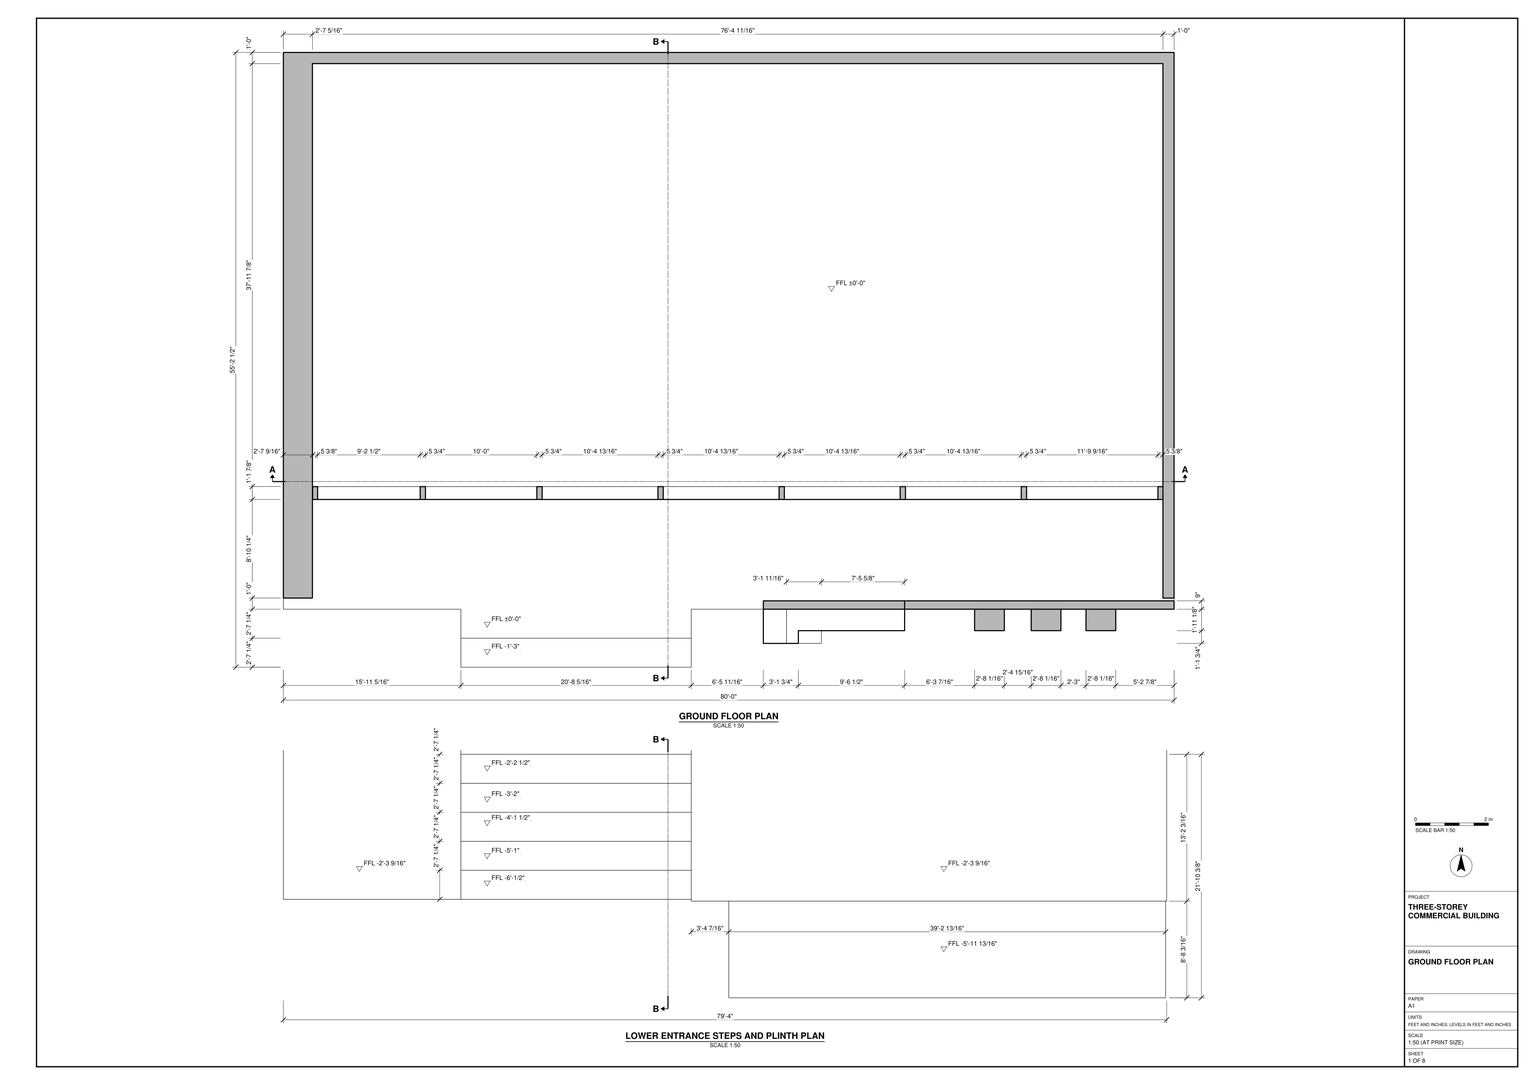
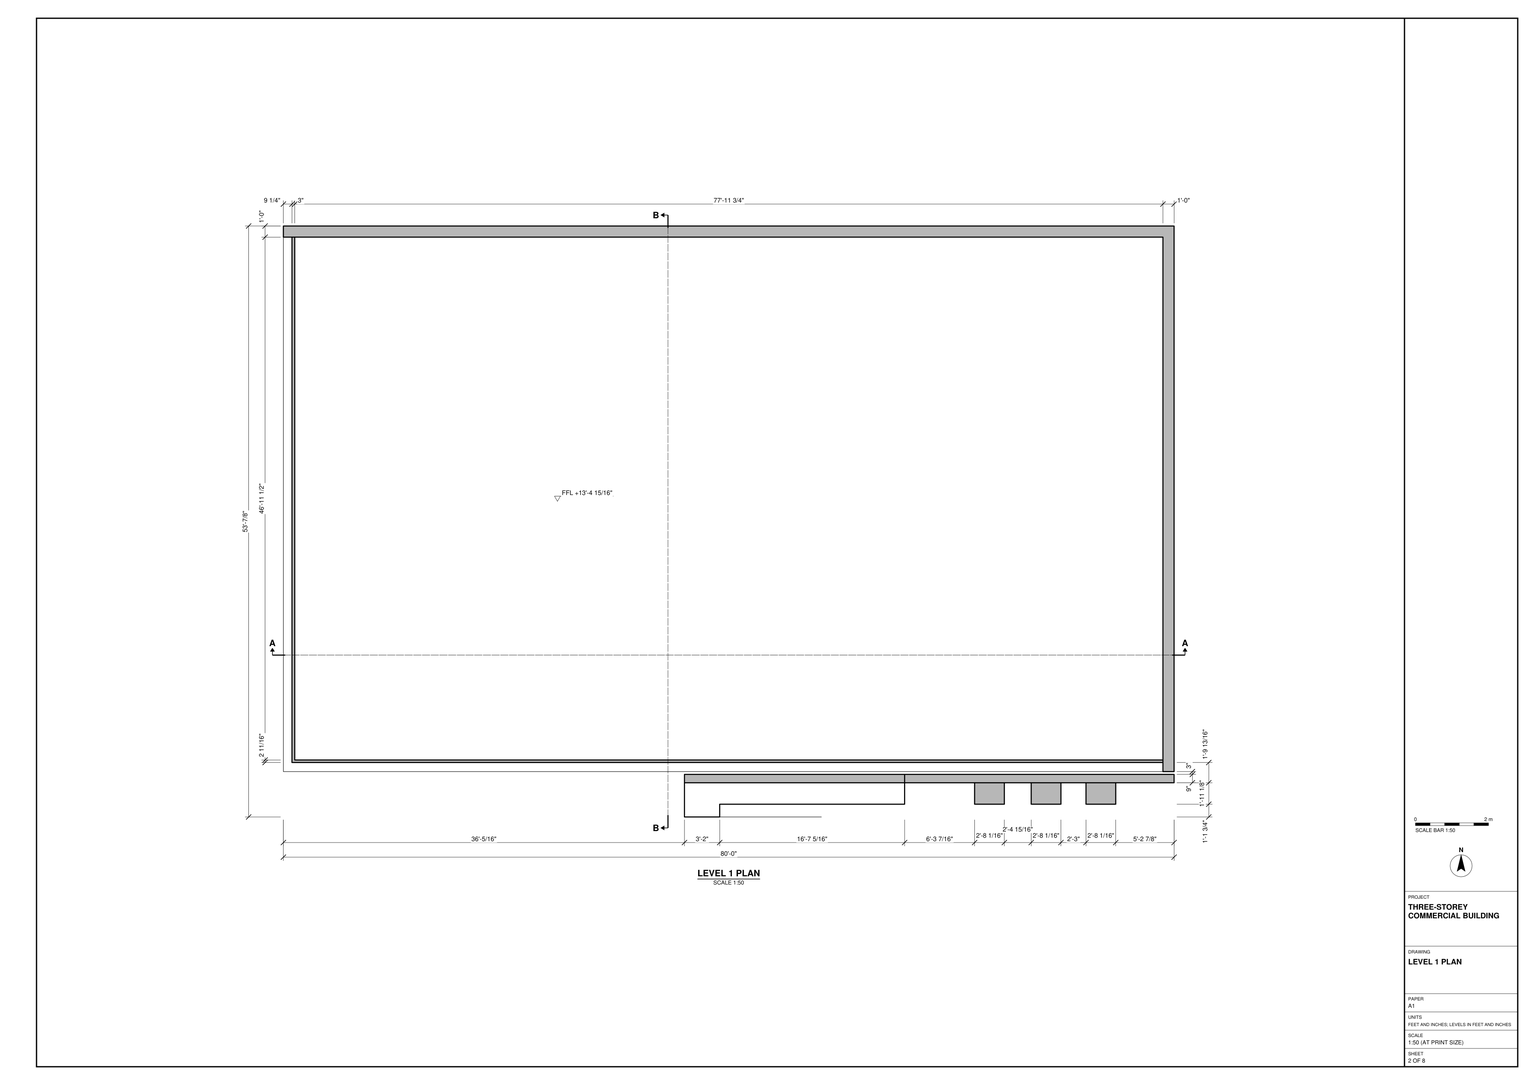
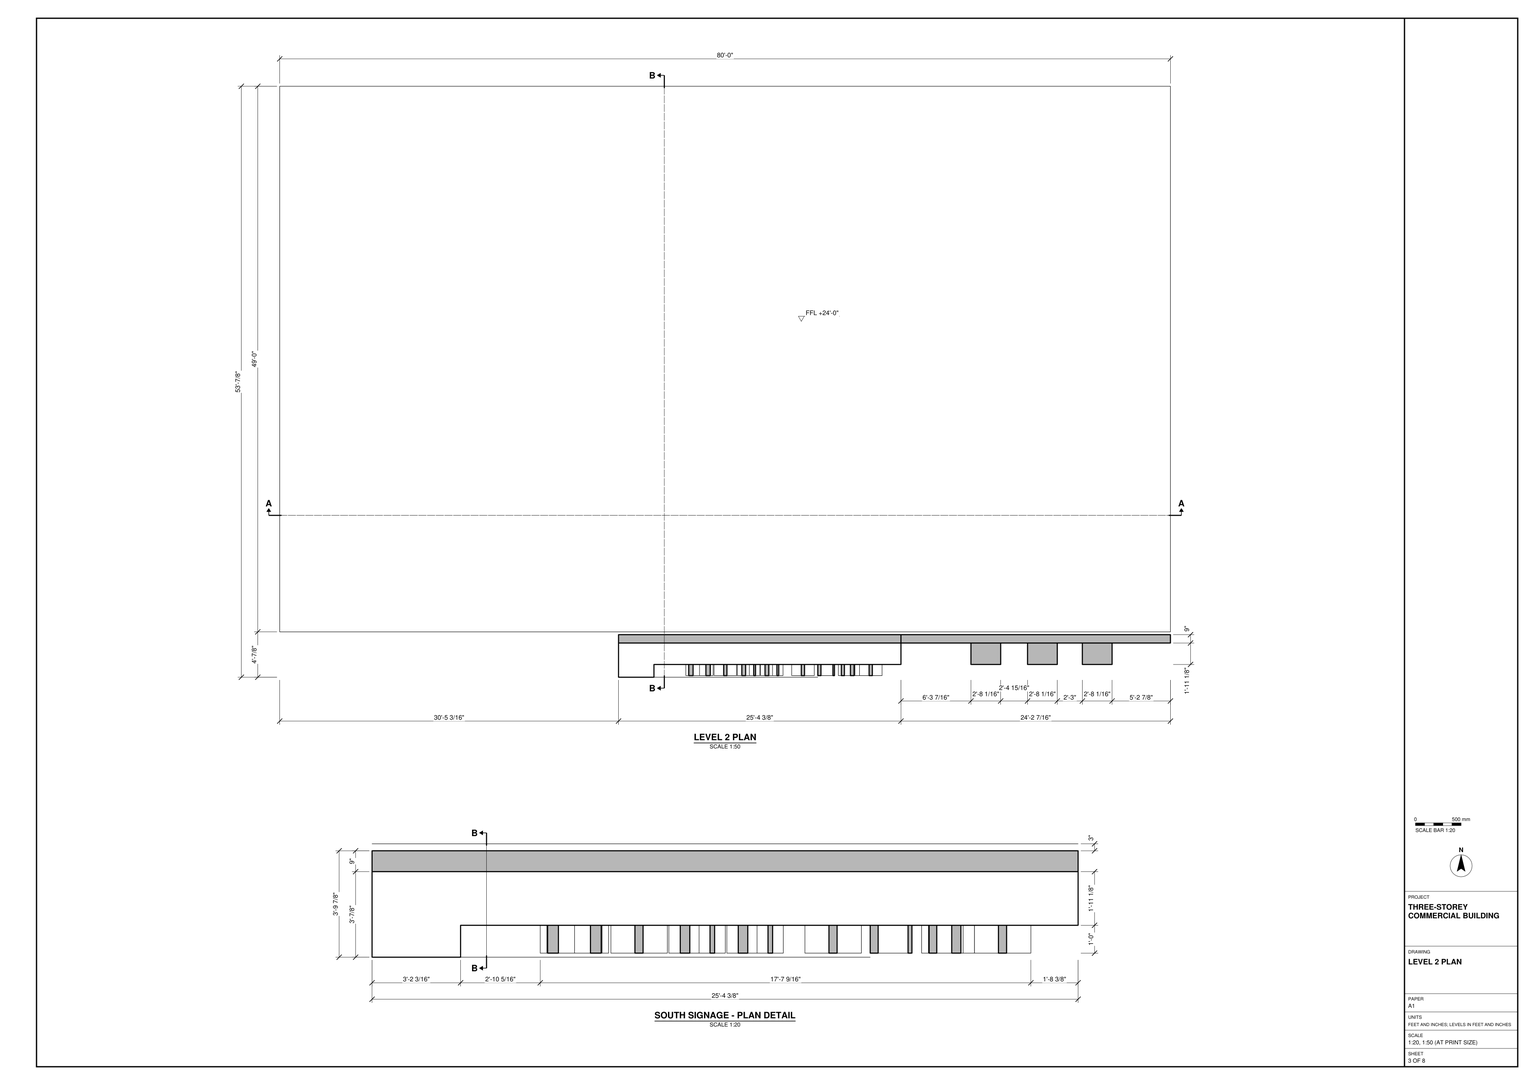
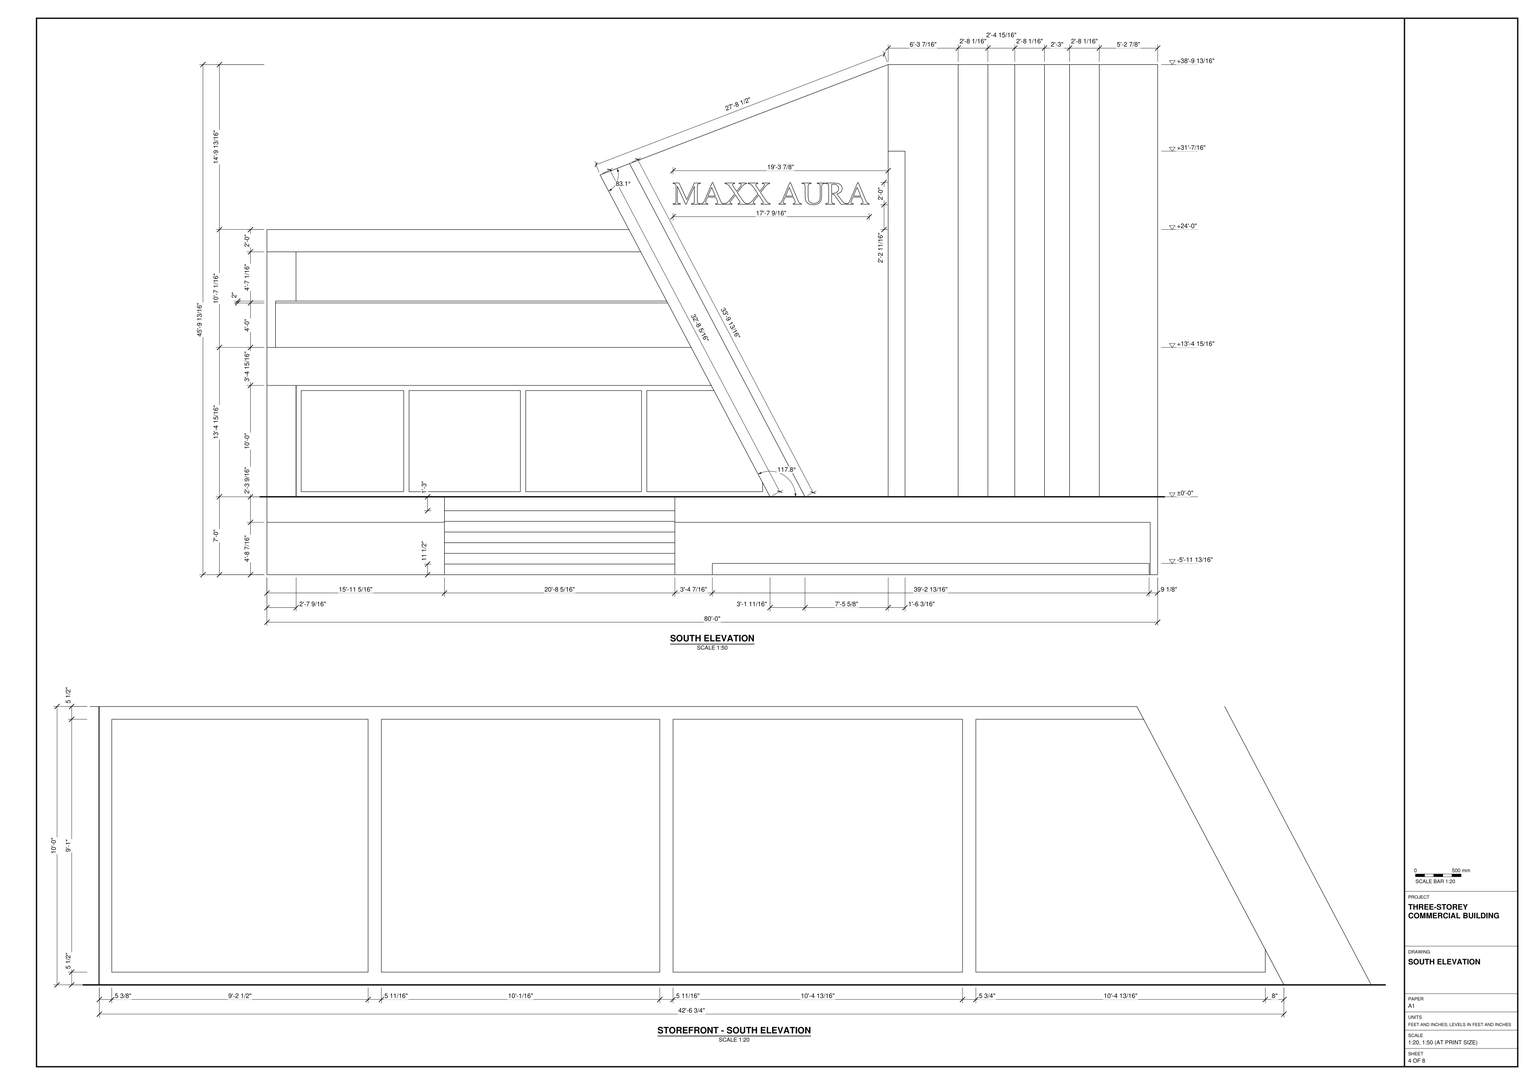
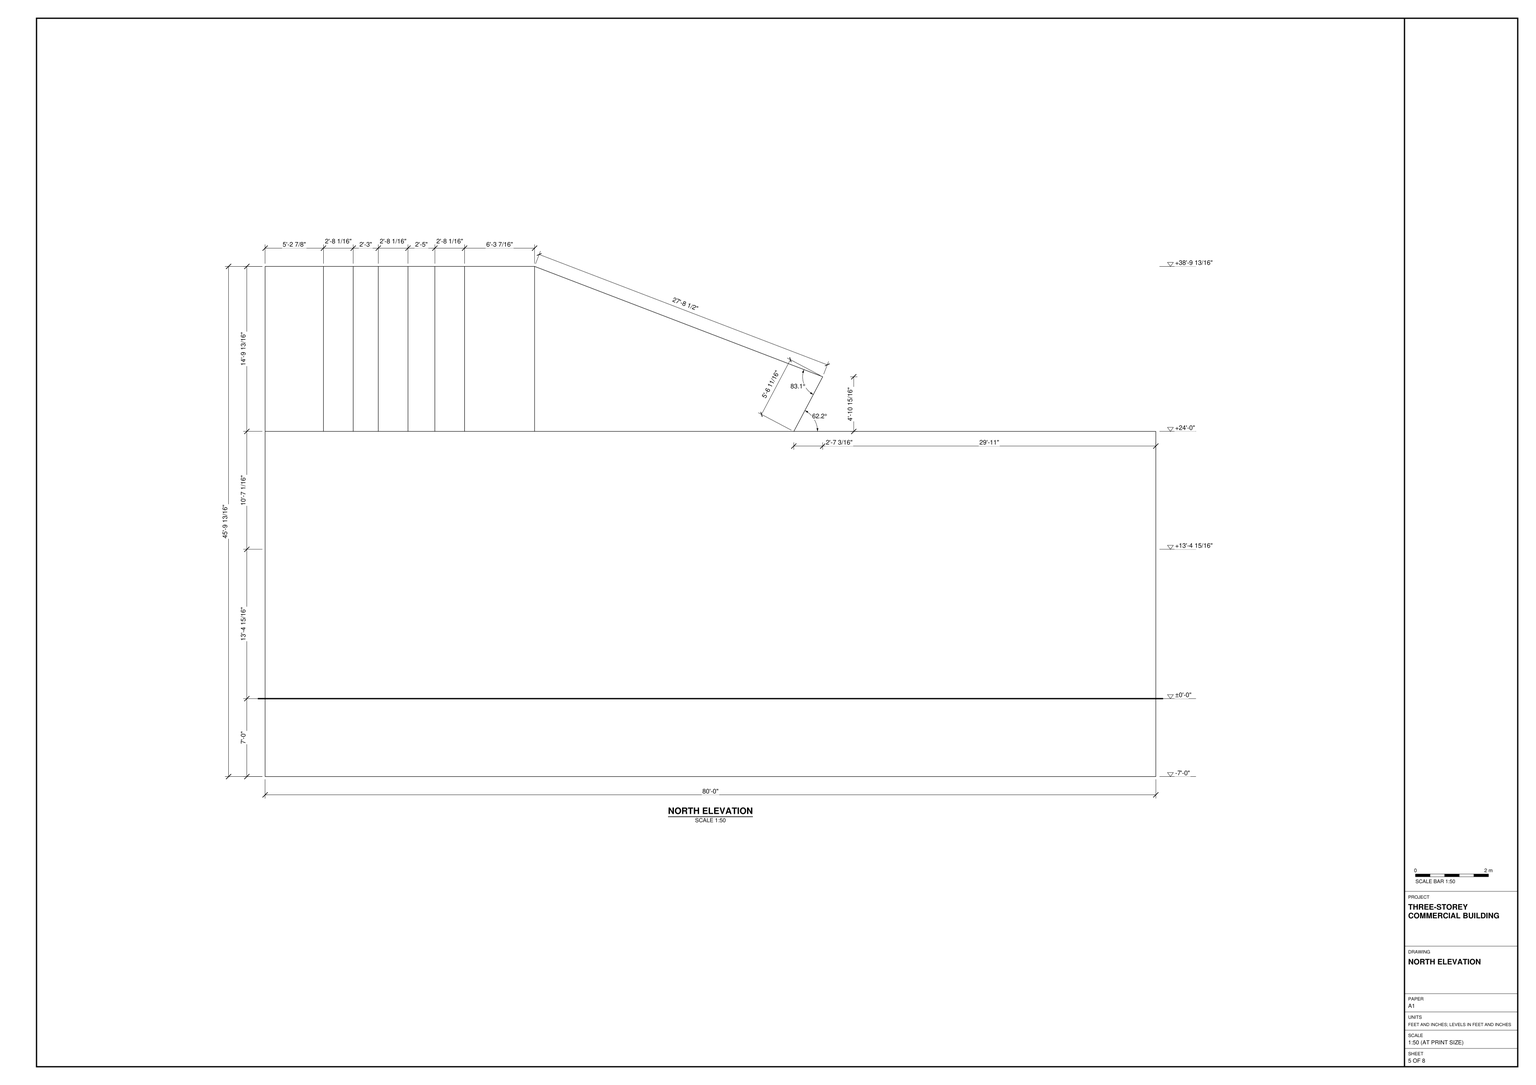
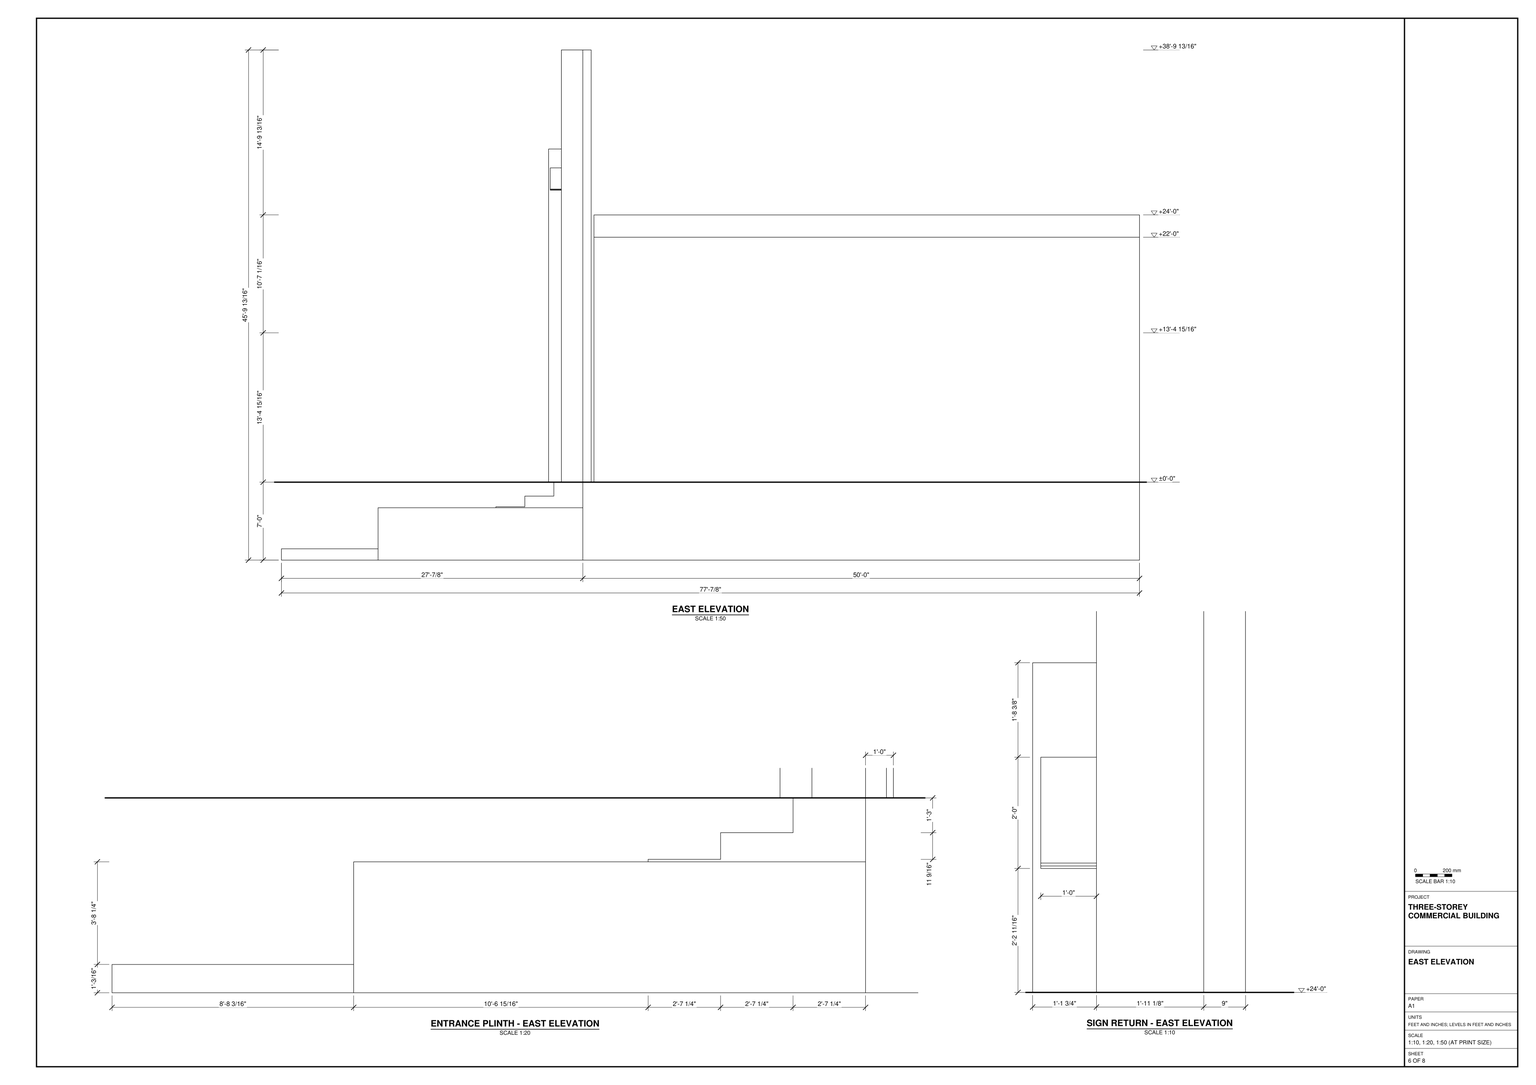
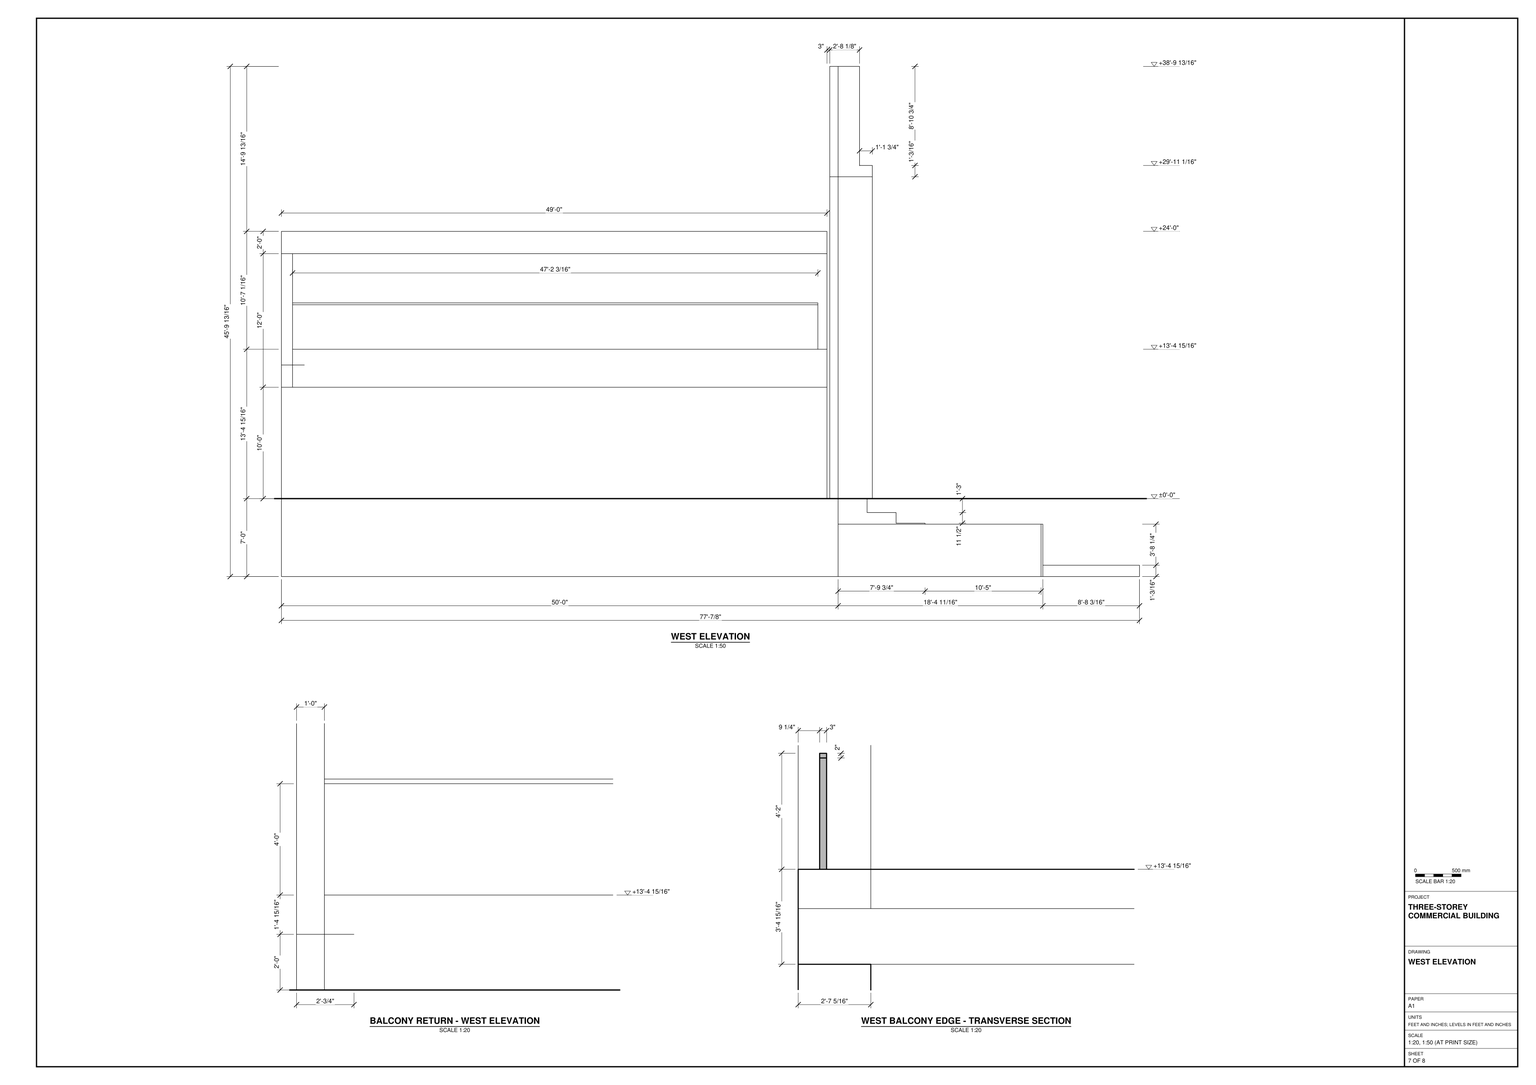
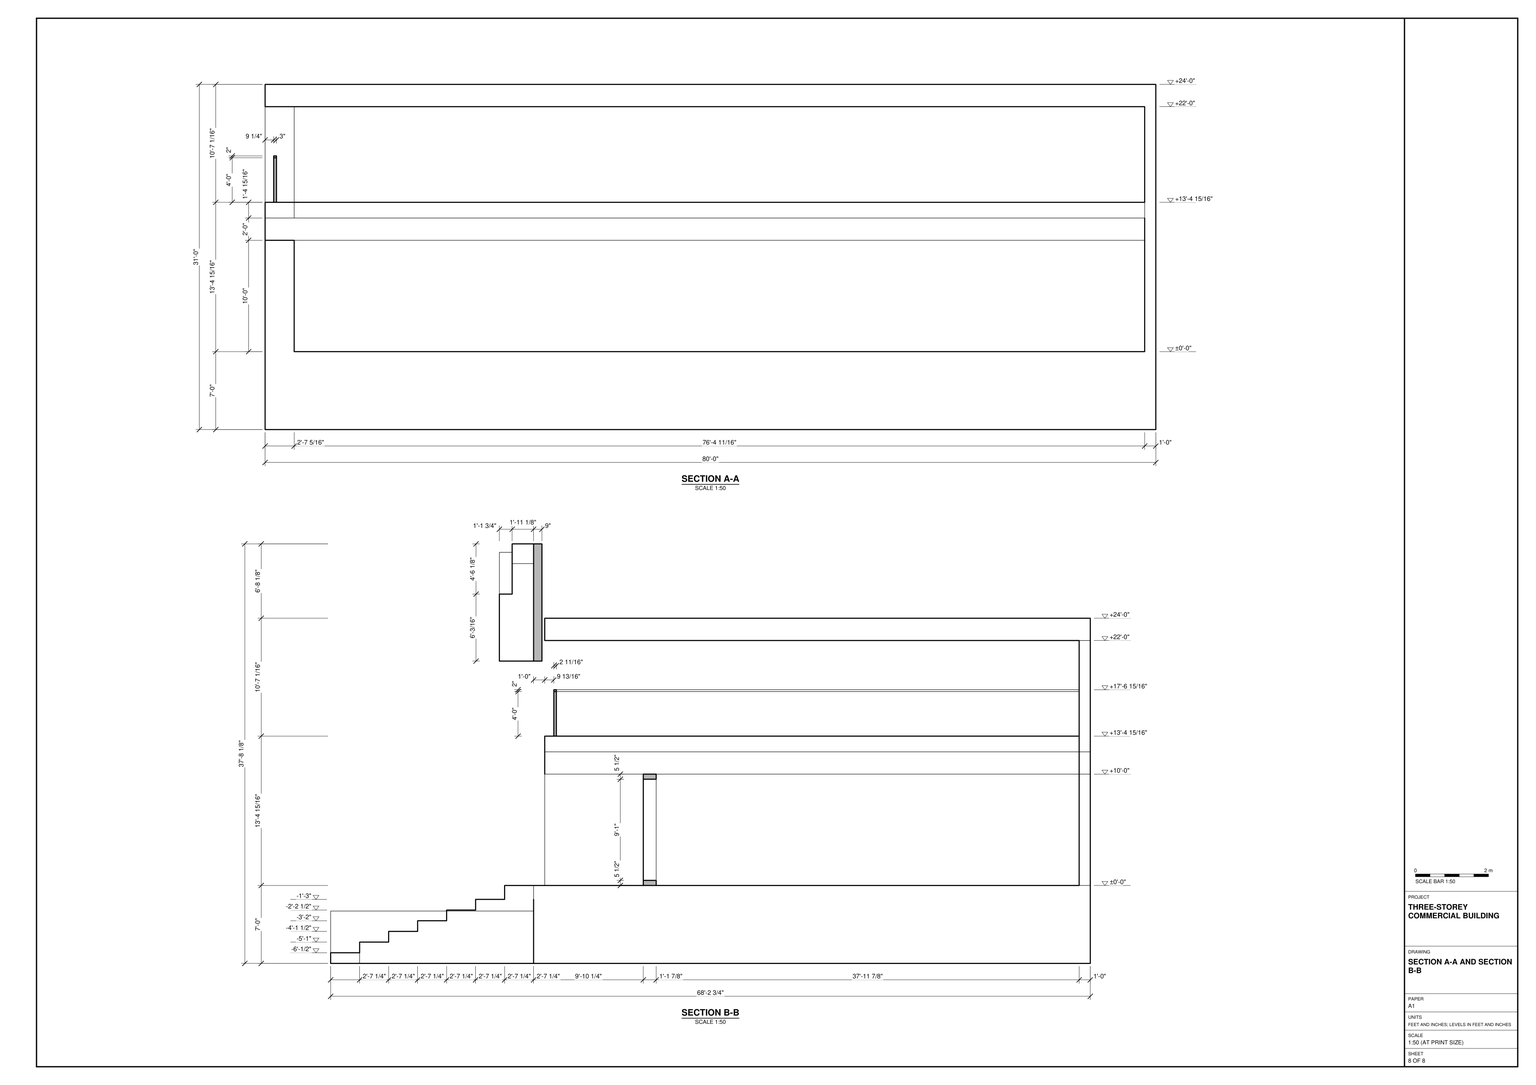
Build the three-storey commercial building in SketchUp from task_files/diagram_01.pdf. Work in feet and inches. Orient the south frontage along the X axis. The complete model, including the entrance steps, plinth and projecting facade elements, is 80'-0" wide, 77'-7/8" deep and 45'-9 13/16" high. Set the finished floor levels to ±0'-0", +13'-4 15/16" and +24'-0".

Model the rectangular floor slabs, perimeter walls and roof using the outlines and thicknesses shown. Keep the floor interiors open as drawn. At ground level, set the row of front openings back from the ends of the side walls and follow the bay spacing on the plan. Use the lower entrance plan to place the broad stair left of centre, with plinth areas to either side and a lower platform extending forward on the right. Model the projections on the right of the south facade and use the enlarged sign detail to set the raised lettering out from its backing.

Keep walls, slabs, roof and stairs in separate groups or components. Treat any furniture or built-in joinery shown as separate pieces and use components for repeated parts. Decor and loose items shown may be represented by any suitable library component. Save one SketchUp model as output_files/three_storey_commercial_building_with_entrance_steps.skp.

# SketchUp Ruby script. Lengths in inches.
U = 1.inch
M = Sketchup.active_model
def pt(a) = Geom::Point3d.new(a.map { |v| v * U })
def face(e, loops, mat)
  f = e.add_face(loops[0].map { |a| pt(a) })
  loops[1..].each { |l| e.add_face(l.map { |a| pt(a) }).erase! }
  f.material = f.back_material = mat if mat
  f
end
# faces: each face lists its corners as indices into pts; further lists are holes
def faces(e, pts, list, mat = nil) = list.each { |f| face(e, (f[0].is_a?(Array) ? f : [f]).map { |l| l.map { |i| pts[i] } }, mat) }
# xy, xz, yz: faces in a plane at the given z, y or x. An outline is a flat list of corners, or four numbers for a rectangle; further outlines are holes
def ring(l) = l.size == 4 ? [[l[0], l[1]], [l[2], l[1]], [l[2], l[3]], [l[0], l[3]]] : l.each_slice(2).to_a
def flat(e, list, mat, &to3) = list.each { |f| face(e, (f[0].is_a?(Array) ? f : [f]).map { |l| ring(l).map { |u, v| to3.(u, v) } }, mat) }
def xy(e, z, list, mat = nil) = flat(e, list, mat) { |x, y| [x, y, z] }
def xz(e, y, list, mat = nil) = flat(e, list, mat) { |x, z| [x, y, z] }
def yz(e, x, list, mat = nil) = flat(e, list, mat) { |y, z| [x, y, z] }
def lines(e, pts, list) = list.each { |a, b| e.add_line(pt(pts[a]), pt(pts[b])) }
# prism: a flat outline (further loops are holes) pulled along v
def prism(e, loops, v, mat = nil)
  f = face(e, loops, mat); d = Geom::Vector3d.new(v.map { |x| x * U })
  f.pushpull(f.normal.samedirection?(d) ? d.length : -d.length)
end
def box(e, o, s, mat = nil) = prism(e, [[o, [o[0] + s[0], o[1], o[2]], [o[0] + s[0], o[1] + s[1], o[2]], [o[0], o[1] + s[1], o[2]]]], [0, 0, s[2]], mat)
def at(x, y, z, deg = 0) = Geom::Transformation.translation(pt([x, y, z])) * Geom::Transformation.rotation(ORIGIN, Z_AXIS, deg.degrees)
def axes(o, x, y, z) = Geom::Transformation.new([*x, 0, *y, 0, *z, 0, *pt(o).to_a, 1])
def part(name) = M.definitions.add(name)
# library, detail: a bought-in or finely detailed component or shape, given as its bounding box
def library(name, o, s) = part(name).tap { |d| box(d.entities, o, s) }
def detail(e, o, s) = box(e.add_group.entities, o, s)
def put(e, d, t, mat = nil) = e.add_instance(d, t).tap { |i| i.material = mat if mat }
def group(e, t, mat = nil) = e.add_group.tap { |g| g.transformation = t; g.material = mat if mat }.entities
root = M.entities
M.materials.add("[Color C08]").color = [102, 51, 0]
M.materials.add("[Color E01]").color = [255, 255, 204]
M.materials.add("[Color M07]").color = [58, 58, 58]
M.materials.add("[Grass Dark Green]").color = [106, 157, 55]
M.materials.add("[Grass Light Green]").color = [138, 158, 69]
M.materials.add("[Metal Embossed]").color = [144, 144, 144]
M.materials.add("[Stone Vein Gray]").color = [166, 165, 165]
M.materials.add("[Translucent Glass Gray]").color = [128, 128, 128]
M.materials["[Translucent Glass Gray]"].alpha = 0.5
c1 = library("MAXX AURA",[0.57,0,0],[211.54,23.98,4])
xy(root,0,[[480.07,0,950.88,104.1875],[439.64,104.1875,952.01,324.875],[0,106.125,191.33,324.875],[191.33,106.125,439.64,137.375],[191.33,137.375,439.64,324.875],
  [0,324.875,960,924.875]])
xy(root,11.5,[[191.33,106.125,439.64,137.375]])
xy(root,12.1875,[[480.07,0,950.88,104.1875]],"[Grass Dark Green]")
xy(root,23,[[191.33,137.375,439.64,168.625]])
xy(root,34.5,[[191.33,168.625,439.64,199.875]])
xy(root,46,[[191.33,199.875,439.64,231.125]])
xy(root,56.4375,[[439.64,104.1875,952.01,324.875],[0,106.125,191.33,324.875]],"[Grass Light Green]")
xy(root,57.5,[[191.33,231.125,439.64,262.375]])
xy(root,69,[[191.33,262.375,439.64,293.625]])
xy(root,84,[[542.26,288,542.26,324.875,669.5625,324.875,669.5625,301.75,579.92,301.75,579.92,288],[191.33,293.625,439.64,293.625,439.64,324.875,542.26,324.875,542.26,333.875,960,333.875,960,336.875,948,336.875,948,912.875,31.3125,912.875,31.3125,336.875,0,336.875,0,324.875,191.33,324.875],[745,301.75,777.0625,324.875],[806,301.75,838.0625,324.875],[865.0625,301.75,897.125,324.875],
  [542.26,324.875,669.5625,333.875],[669.5625,324.875,745,333.875],[745,324.875,777.0625,333.875],[777.0625,324.875,806,333.875],[806,324.875,838.0625,333.875],
  [838.0625,324.875,865.0625,333.875],[865.0625,324.875,897.125,333.875],[897.125,324.875,960,333.875]])
xy(root,204,[[0,336.875,31.3125,912.875]])
xy(root,244.9375,[[0,336.875,948,336.875,948,346.6875,9.25,346.6875,9.25,912.875,0,912.875],[9.25,346.6875,9.25,912.875,12.25,912.875,12.25,349.41,948,349.41,948,346.6875],[12.25,349.41,948,912.875]])
xy(root,292.9375,[[9.25,346.6875,9.25,912.875,12.25,912.875,12.25,349.41,948,349.41,948,346.6875]])
xy(root,294.9375,[[9.25,346.6875,948,346.6875,948,349.41,12.25,349.41,12.25,912.875,9.25,912.875]],"[Metal Embossed]")
xy(root,348,[[0,336.875,948,912.875]])
xy(root,372,[[0,336.875,960,924.875]],"[Color M07]")
xy(root,549.8125,[[745,301.75,777.0625,324.875],[806,301.75,838.0625,324.875],[865.0625,301.75,897.125,324.875],[669.5625,324.875,960,333.875]],"[Color E01]")
xz(root,0,[[480.07,0,950.88,12.1875]],"[Stone Vein Gray]")
xz(root,104.1875,[[480.07,0,950.88,12.1875]])
xz(root,104.1875,[[439.64,0,480.07,0,480.07,12.1875,950.88,12.1875,950.88,0,952.01,0,952.01,56.4375,439.64,56.4375]],"[Stone Vein Gray]")
xz(root,106.125,[[191.33,0,439.64,11.5]])
xz(root,106.125,[[0,0,191.33,56.4375]],"[Stone Vein Gray]")
xz(root,137.375,[[191.33,11.5,439.64,23]])
xz(root,168.625,[[191.33,23,439.64,34.5]])
xz(root,199.875,[[191.33,34.5,439.64,46]])
xz(root,231.125,[[191.33,46,439.64,57.5]])
xz(root,262.375,[[191.33,57.5,439.64,69]])
xz(root,288,[[542.26,84,579.92,84,390.8,443.05,359.03,430.88]],"[Color E01]")
xz(root,293.625,[[191.33,69,439.64,84]])
xz(root,301.75,[[579.92,84,669.5625,84,669.5625,549.8125,390.8,443.05],[745,84,777.0625,549.8125],[806,84,838.0625,549.8125],[865.0625,84,897.125,549.8125]],"[Color E01]")
xz(root,324.875,[[0,0,191.33,56.4375],[191.33,0,439.64,69],[439.64,0,952.01,56.4375],[542.26,84,669.5625,84,669.5625,549.8125,359.03,430.88],[745,84,777.0625,549.8125],
  [806,84,838.0625,549.8125],[865.0625,84,897.125,549.8125]])
xz(root,324.875,[[952.01,0,960,0,960,84,439.64,84,439.64,56.4375,952.01,56.4375],[0,56.4375,191.33,84],[687.75,84,745,84,745,549.8125,669.5625,549.8125,669.5625,456.47,687.75,456.47],[777.0625,84,806,549.8125],[838.0625,84,865.0625,549.8125],
  [897.125,84,960,549.8125]],"[Color E01]")
xz(root,324.875,[[669.5625,84,687.75,456.47]],"[Color M07]")
xz(root,333.875,[[542.26,84,359.03,430.88,669.5625,549.8125,669.5625,84],[669.5625,84,745,549.8125],[745,84,777.0625,549.8125],[777.0625,84,806,549.8125],[806,84,838.0625,549.8125],
  [838.0625,84,865.0625,549.8125],[865.0625,84,897.125,549.8125],[897.125,84,960,549.8125]],"[Color E01]")
xz(root,336.875,[[948,84,960,204],[948,204,960,228],[948,228,960,348],[948,348,960,372]])
xz(root,336.875,[[0,84,31.3125,204],[0,204,948,244.9375]],"[Color E01]")
xz(root,336.875,[[0,348,948,372]],"[Color M07]")
xz(root,346.6875,[[9.25,292.9375,948,294.9375]],"[Metal Embossed]")
xz(root,346.6875,[[9.25,244.9375,948,292.9375]],"[Translucent Glass Gray]")
xz(root,349.41,[[12.25,292.9375,948,294.9375]],"[Metal Embossed]")
xz(root,349.41,[[12.25,244.9375,948,292.9375]],"[Translucent Glass Gray]")
xz(root,912.875,[[31.3125,84,948,204],[0,204,948,228],[0,228,31.3125,244.9375],[31.3125,228,948,244.9375],[9.25,244.9375,12.25,292.9375],
  [9.25,292.9375,12.25,294.9375]])
xz(root,912.875,[[0,244.9375,0,348,31.3125,348,31.3125,244.9375,12.25,244.9375,12.25,294.9375,9.25,294.9375,9.25,244.9375],[31.3125,244.9375,948,348]],"[Color E01]")
xz(root,924.875,[[0,0,960,372]],"[Color E01]")
yz(root,0,[[324.875,0,924.875,84],[336.875,84,924.875,204],[336.875,204,912.875,244.9375],[912.875,204,924.875,228],[912.875,228,924.875,348]],"[Color E01]")
yz(root,0,[[336.875,348,924.875,372]],"[Color M07]")
yz(root,0,[[106.125,0,324.875,56.4375]],"[Stone Vein Gray]")
yz(root,9.25,[[346.6875,292.9375,912.875,294.9375]],"[Metal Embossed]")
yz(root,9.25,[[346.6875,244.9375,912.875,292.9375]],"[Translucent Glass Gray]")
yz(root,12.25,[[349.41,292.9375,912.875,294.9375]],"[Metal Embossed]")
yz(root,12.25,[[349.41,244.9375,912.875,292.9375]],"[Translucent Glass Gray]")
yz(root,31.3125,[[336.875,84,912.875,204]])
yz(root,191.33,[[106.125,0,137.375,11.5],[137.375,0,137.375,23,168.625,23,168.625,34.5,199.875,34.5,199.875,46,231.125,46,231.125,56.4375,324.875,56.4375,324.875,0],[231.125,56.4375,231.125,57.5,262.375,57.5,262.375,69,293.625,69,293.625,84,324.875,84,324.875,56.4375]])
yz(root,191.33,[[106.125,11.5,137.375,11.5,137.375,23,168.625,23,168.625,34.5,199.875,34.5,199.875,46,231.125,46,231.125,56.4375,106.125,56.4375]],"[Stone Vein Gray]")
yz(root,439.64,[[104.1875,0,106.125,56.4375],[106.125,0,137.375,11.5],[137.375,0,324.875,0,324.875,56.4375,231.125,56.4375,231.125,46,199.875,46,199.875,34.5,168.625,34.5,168.625,23,137.375,23],[231.125,56.4375,324.875,56.4375,324.875,84,293.625,84,293.625,69,262.375,69,262.375,57.5,231.125,57.5]])
yz(root,439.64,[[106.125,11.5,106.125,56.4375,231.125,56.4375,231.125,46,199.875,46,199.875,34.5,168.625,34.5,168.625,23,137.375,23,137.375,11.5]],"[Stone Vein Gray]")
yz(root,480.07,[[0,0,104.1875,12.1875]],"[Stone Vein Gray]")
yz(root,669.5625,[[324.875,84,333.875,549.8125]])
yz(root,669.5625,[[301.75,84,324.875,549.8125]],"[Color E01]")
yz(root,745,[[301.75,84,324.875,549.8125]],"[Color E01]")
yz(root,777.0625,[[301.75,84,324.875,549.8125]],"[Color E01]")
yz(root,806,[[301.75,84,324.875,549.8125]],"[Color E01]")
yz(root,838.0625,[[301.75,84,324.875,549.8125]],"[Color E01]")
yz(root,865.0625,[[301.75,84,324.875,549.8125]],"[Color E01]")
yz(root,897.125,[[301.75,84,324.875,549.8125]],"[Color E01]")
yz(root,948,[[336.875,84,912.875,228],[346.6875,244.9375,349.41,292.9375],[346.6875,292.9375,349.41,294.9375]])
yz(root,948,[[336.875,244.9375,336.875,348,912.875,348,912.875,244.9375,349.41,244.9375,349.41,294.9375,346.6875,294.9375,346.6875,244.9375]],"[Color E01]")
yz(root,950.88,[[0,0,104.1875,12.1875]],"[Stone Vein Gray]")
yz(root,952.01,[[104.1875,0,324.875,56.4375]],"[Stone Vein Gray]")
yz(root,960,[[324.875,0,924.875,84],[324.875,84,333.875,549.8125],[336.875,84,924.875,348]],"[Color E01]")
yz(root,960,[[336.875,348,924.875,372]],"[Color M07]")
p = [[359.03,324.875,430.88],[542.26,324.875,84],[542.26,288,84],[359.03,288,430.88],[579.92,301.75,84],[390.8,301.75,443.05],
  [390.8,288,443.05],[579.92,288,84],[359.03,333.875,430.88],[542.26,333.875,84],[669.5625,324.875,549.8125],[669.5625,301.75,549.8125],
  [669.5625,333.875,549.8125],[31.3125,912.875,228],[31.3125,336.875,228],[0,900.125,228],[0,912.875,228],[191.33,168.625,11.5],
  [439.64,168.625,11.5],[191.33,199.875,23],[439.64,199.875,23],[191.33,231.125,34.5],[439.64,231.125,34.5],[191.33,262.375,46],
  [439.64,262.375,46],[191.33,293.625,57.5],[439.64,293.625,57.5]]
faces(root,p,[[0,1,2,3],[4,5,6,7],[1,0,8,9],[10,0,3,6,5,11],[0,10,12,8]],"[Color E01]")
lines(root,p,[[13,14],[15,16],[17,18],[19,20],[21,22],[23,24],[25,26]])
put(root,c1,axes([437.1,301.75,398.71],[1,0,0],[0,0,1],[0,-3,0]),"[Color M07]")
g1 = group(root,at(31.55,443.11,84))
xy(g1,0,[[0,0,916.45,13.875]])
xy(g1,5.5,[[5.38,0,115.88,13.875],[121.61,0,241.64,13.875],[247.37,0,372.17,13.875],[377.9,0,502.7,13.875],[508.42,0,633.23,13.875],
  [638.95,0,763.75,13.875],[769.48,0,911.07,13.875]],"[Color C08]")
xy(g1,114.5,[[5.38,0,115.88,13.875],[121.61,0,241.64,13.875],[247.37,0,372.17,13.875],[377.9,0,502.7,13.875],[508.42,0,633.23,13.875],
  [638.95,0,763.75,13.875],[769.48,0,911.07,13.875]])
xy(g1,120,[[0,0,916.45,13.875]],"[Color C08]")
xz(g1,0,[[[0,0,916.45,120],[769.48,5.5,911.07,114.5],[247.37,5.5,372.17,114.5],[377.9,5.5,502.7,114.5],[508.42,5.5,633.23,114.5],[638.95,5.5,763.75,114.5],[121.61,5.5,241.64,114.5],[5.38,5.5,115.88,114.5]]],"[Color C08]")
xz(g1,0,[[5.38,5.5,115.88,114.5],[121.61,5.5,241.64,114.5],[247.37,5.5,372.17,114.5],[377.9,5.5,502.7,114.5],[508.42,5.5,633.23,114.5],
  [638.95,5.5,763.75,114.5],[769.48,5.5,911.07,114.5]],"[Translucent Glass Gray]")
xz(g1,13.875,[[[0,0,916.45,120],[769.48,5.5,911.07,114.5],[247.37,5.5,372.17,114.5],[377.9,5.5,502.7,114.5],[508.42,5.5,633.23,114.5],[638.95,5.5,763.75,114.5],[121.61,5.5,241.64,114.5],[5.38,5.5,115.88,114.5]]],"[Color C08]")
yz(g1,0,[[0,0,13.875,120]],"[Color C08]")
yz(g1,5.38,[[0,5.5,13.875,114.5]],"[Color C08]")
yz(g1,115.88,[[0,5.5,13.875,114.5]],"[Color C08]")
yz(g1,121.61,[[0,5.5,13.875,114.5]],"[Color C08]")
yz(g1,241.64,[[0,5.5,13.875,114.5]],"[Color C08]")
yz(g1,247.37,[[0,5.5,13.875,114.5]],"[Color C08]")
yz(g1,372.17,[[0,5.5,13.875,114.5]],"[Color C08]")
yz(g1,377.9,[[0,5.5,13.875,114.5]],"[Color C08]")
yz(g1,502.7,[[0,5.5,13.875,114.5]],"[Color C08]")
yz(g1,508.42,[[0,5.5,13.875,114.5]],"[Color C08]")
yz(g1,633.23,[[0,5.5,13.875,114.5]],"[Color C08]")
yz(g1,638.95,[[0,5.5,13.875,114.5]],"[Color C08]")
yz(g1,763.75,[[0,5.5,13.875,114.5]],"[Color C08]")
yz(g1,769.48,[[0,5.5,13.875,114.5]],"[Color C08]")
yz(g1,911.07,[[0,5.5,13.875,114.5]],"[Color C08]")
yz(g1,916.45,[[0,0,13.875,120]],"[Color C08]")
